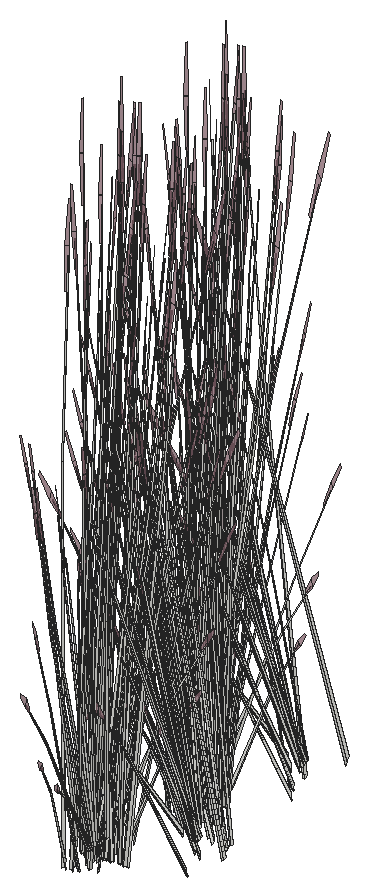
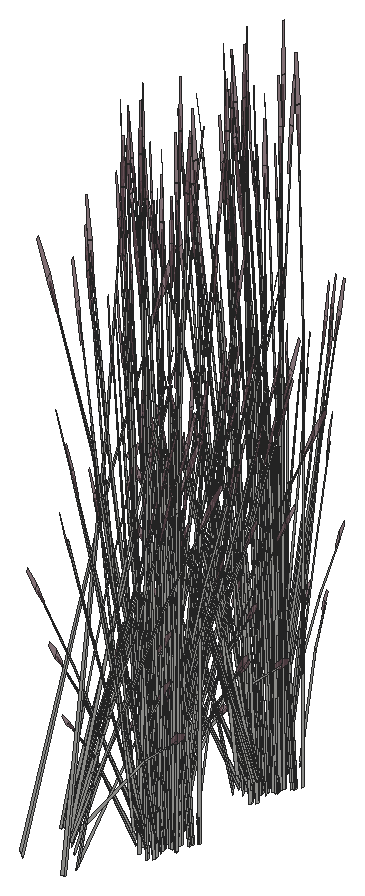
# SketchUp Ruby script. Lengths in inches.
U = 1.inch
M = Sketchup.active_model
def pt(a) = Geom::Point3d.new(a.map { |v| v * U })
def face(e, loops, mat)
  f = e.add_face(loops[0].map { |a| pt(a) })
  loops[1..].each { |l| e.add_face(l.map { |a| pt(a) }).erase! }
  f.material = f.back_material = mat if mat
  f
end
# faces: each face lists its corners as indices into pts; further lists are holes
def faces(e, pts, list, mat = nil) = list.each { |f| face(e, (f[0].is_a?(Array) ? f : [f]).map { |l| l.map { |i| pts[i] } }, mat) }
# xy, xz, yz: faces in a plane at the given z, y or x. An outline is a flat list of corners, or four numbers for a rectangle; further outlines are holes
def ring(l) = l.size == 4 ? [[l[0], l[1]], [l[2], l[1]], [l[2], l[3]], [l[0], l[3]]] : l.each_slice(2).to_a
def flat(e, list, mat, &to3) = list.each { |f| face(e, (f[0].is_a?(Array) ? f : [f]).map { |l| ring(l).map { |u, v| to3.(u, v) } }, mat) }
def xy(e, z, list, mat = nil) = flat(e, list, mat) { |x, y| [x, y, z] }
def xz(e, y, list, mat = nil) = flat(e, list, mat) { |x, z| [x, y, z] }
def yz(e, x, list, mat = nil) = flat(e, list, mat) { |y, z| [x, y, z] }
def lines(e, pts, list) = list.each { |a, b| e.add_line(pt(pts[a]), pt(pts[b])) }
# prism: a flat outline (further loops are holes) pulled along v
def prism(e, loops, v, mat = nil)
  f = face(e, loops, mat); d = Geom::Vector3d.new(v.map { |x| x * U })
  f.pushpull(f.normal.samedirection?(d) ? d.length : -d.length)
end
def box(e, o, s, mat = nil) = prism(e, [[o, [o[0] + s[0], o[1], o[2]], [o[0] + s[0], o[1] + s[1], o[2]], [o[0], o[1] + s[1], o[2]]]], [0, 0, s[2]], mat)
def at(x, y, z, deg = 0) = Geom::Transformation.translation(pt([x, y, z])) * Geom::Transformation.rotation(ORIGIN, Z_AXIS, deg.degrees)
def axes(o, x, y, z) = Geom::Transformation.new([*x, 0, *y, 0, *z, 0, *pt(o).to_a, 1])
def part(name) = M.definitions.add(name)
# library, detail: a bought-in or finely detailed component or shape, given as its bounding box
def library(name, o, s) = part(name).tap { |d| box(d.entities, o, s) }
def detail(e, o, s) = box(e.add_group.entities, o, s)
def put(e, d, t, mat = nil) = e.add_instance(d, t).tap { |i| i.material = mat if mat }
def group(e, t, mat = nil) = e.add_group.tap { |g| g.transformation = t; g.material = mat if mat }.entities
root = M.entities
M.materials.add("LightPink_Translucent").color = [144, 107, 117]
M.materials["LightPink_Translucent"].alpha = 0.75
c1 = part("blade")
p = [[2.15,0.21,22],[0,0.17,0],[0.09,0.45,0],[2.18,0.31,22],[2.29,0.31,22],[0.38,0.45,0],
  [2.48,0.24,33],[2.49,0.24,33],[2.48,0.22,33]]
faces(c1.entities,p,[[0,1,2,3],[4,5,2,3],[6,3,4,7],[8,0,3,6]])
c2 = part("seeds")
p = [[0.3,-0.1,1.38],[-0.01,-0.03,1.59],[-0.01,-0.03,0.03],[0.14,-0.07,-0.07],[0.29,-0.03,3],[0.15,0.01,3.11]]
faces(c2.entities,p,[[0,1,2,3],[1,0,4,5]],"LightPink_Translucent")
c3 = part("blade with seeds")
put(c3.entities,c1,at(0,0,0))
put(c3.entities,c2,axes([2.4,0.25,30.99],[1.5799,-0.05474,1.17369],[-0.12525,1.92788,0.29478],[-0.07173,-0.02425,1.56792]))
put(root,c3,axes([404.3,9.67,-9.59],[-0.14537,0.11002,1.33163],[-0.43536,-0.19256,-0.28638],[0.0807,-0.23948,0.56934]))
put(root,c3,axes([404.65,10.49,-7.36],[0.01331,-0.50278,-0.66157],[0.56035,0.03377,0.07984],[0.05914,-0.213,0.93586]))
put(root,c3,axes([405.43,9.7,-7.61],[-0.00494,-0.10818,1.62908],[-0.41695,-0.31265,-0.25764],[0.06446,-0.18952,0.13065]))
put(root,c3,axes([404.02,10.23,-8.39],[-0.09522,0.18683,1.59586],[-0.39947,-0.38663,0.12904],[0.18021,-0.24097,0.68222]))
put(root,c3,axes([405.32,9.32,-7.62],[-0.05194,0.04152,1.65179],[-0.50886,-0.14007,-0.15608],[-0.01842,-0.18118,0.29231]))
put(root,c3,axes([403.76,8.8,-9.42],[0.06561,0.31695,1.06958],[-0.36394,-0.17555,0.78586],[0.03916,-0.16229,0.23558]))
put(root,c3,axes([404.54,10.32,-7.64],[-0.3661,-0.36521,-0.47583],[0.38674,-0.31985,-0.36857],[0.0557,-0.18556,0.91046]))
put(root,c3,axes([403.74,9.78,-7.59],[0.50393,0.1421,0.447],[-0.17232,0.46717,0.36857],[-0.03028,-0.18372,0.92496]))
put(root,c3,axes([404.92,10.51,-7.3125],[-0.56206,-0.02693,-0.11324],[0.01536,-0.50991,-0.62851],[0.03904,-0.19638,0.95501]))
put(root,c3,axes([404.88,10.1875,-7.78],[0.34603,-0.28618,-0.32977],[0.32756,0.32677,0.42575],[0.04984,-0.16603,0.81462]))
put(root,c3,axes([404.88,10.3,-7.59],[0.36417,0.37086,0.447],[-0.38674,0.31985,0.36857],[0.06718,-0.174,0.92496]))
put(root,c3,axes([405.01,10.33,-7.6],[0.42027,0.02533,0.05988],[-0.01152,0.38243,0.47138],[0.04398,-0.14649,0.71878]))
put(root,c3,axes([404.7,10.59,-7.3],[-0.34603,0.28618,0.32977],[-0.32756,-0.32677,-0.42575],[0.04984,-0.16603,0.81462]))
put(root,c3,axes([402.42,10.12,-9.79],[-0.31974,-0.54466,0],[0.53494,-0.30375,-0.48057],[0.12184,-0.06918,1.52448]))
put(root,c3,axes([402.86,10.03,-10.12],[0.47863,-0.27177,-0.46235],[0.28609,0.48733,0],[0.10901,-0.0619,1.46668]))
put(root,c3,axes([403.42,11.15,-10.08],[0.34446,-0.40855,-0.58063],[0.42791,0.37046,-0.15239],[0.13803,-0.10191,1.28164]))
put(root,c3,axes([403.05,11.62,-9.52],[-0.05959,-0.62022,-0.27094],[0.62068,-0.0375,-0.46562],[0.1093,-0.08261,1.4872]))
put(root,c3,axes([405.3,11.48,-7.3],[-0.44516,0.07768,0.32977],[-0.11755,-0.44407,-0.42575],[0.12757,-0.11927,0.81462]))
put(root,c3,axes([402.97,10.25,-10.11],[0.47712,0.13449,-0.28847],[-0.12013,0.47362,0.28847],[0.09619,-0.05462,1.29413]))
put(root,c3,axes([403.13,12.1,-9.73],[0.57623,0.26344,0.22409],[-0.27732,0.5474,0.46562],[0,-0.12618,1.49497]))
put(root,c3,axes([402.95,11.74,-9.47],[-0.55535,0.03355,0.41661],[-0.05022,-0.55698,-0.2005],[0.09942,-0.05645,1.33761]))
put(root,c3,axes([403.73,11.99,-9.95],[0,-0.62892,0],[0.63949,0,0],[0,0,1.6711]))
put(root,c3,axes([404.5,10.54,-9.69],[-0.47863,-0.27177,0.46235],[0.28609,-0.48733,0],[0.10901,0.0619,1.46668]))
put(root,c3,axes([403.42,11.59,-9.8],[-0.42403,0.49328,0.42607],[-0.50377,-0.43543,0.16719],[0.10223,-0.04923,1.47927]))
put(root,c3,axes([402.6875,10.78,-9.7],[-0.14774,0.54019,0.16428],[-0.54062,-0.15287,0.32672],[0.09339,-0.00263,1.49371]))
put(root,c3,axes([403.82,11.38,-9.5625],[0.09866,-0.48509,0.13483],[0.48202,0.0842,-0.38503],[0.08772,0.04981,1.18024]))
put(root,c3,axes([403.61,11.51,-9.47],[-0.30722,-0.45622,0.41661],[0.46535,-0.32126,-0.2005],[0.09942,0.05645,1.33761]))
put(root,c3,axes([403.77,11.54,-9.52],[0.51635,-0.36087,-0.27094],[0.34336,0.5099,-0.46562],[0.1274,0.05178,1.4872]))
put(root,c3,axes([410.18,15.48,-7.36],[-0.43608,-0.26272,-0.66157],[0.30991,-0.46038,0.07984],[-0.158,-0.15687,0.93586]))
put(root,c3,axes([404.16,12.13,-9.95],[0.57217,0,0],[0,0.56272,0],[0,0,1.66132]))
put(root,c3,axes([404.32,10.8125,-9.7],[-0.54955,0.14427,0.16428],[-0.1357,-0.53689,0.32672],[0.04901,0.07823,1.49371]))
put(root,c3,axes([404.9375,10.78,-10.11],[0.12013,0.47362,-0.28847],[-0.47712,0.13449,0.28847],[0.09619,0.05462,1.29413]))
put(root,c3,axes([409.32,15.04,-10.61],[-0.04954,0.0716,1.6421],[-0.50062,0.15438,-0.25086],[-0.12094,-0.14044,0.2797]))
put(root,c3,axes([403.98,11.84,-9.78],[-0.64638,-0.11452,0.45814],[0.13155,-0.64678,0.17978],[0.09446,0.06245,1.59061]))
put(root,c3,axes([409.06,15.77,-8.39],[0.18996,0.09365,1.59586],[-0.39312,0.39287,0.12904],[-0.24502,-0.17723,0.68222]))
put(root,c3,axes([404.08,13.375,-9.97],[0.53691,-0.18442,-0.17877],[0.18866,0.53125,0.00007],[0.05927,-0.02038,1.61933]))
put(root,c3,axes([404.15,12.37,-9.9375],[0.35699,0.35109,0],[-0.35699,0.35109,0],[0,0,1.57621]))
put(root,c3,axes([405.11,12.22,-9.7],[-0.40181,-0.39593,0.16428],[0.40492,-0.38402,0.32672],[-0.04438,0.08086,1.49371]))
put(root,c3,axes([409.97,15.49,-7.64],[-0.50465,0.12921,-0.47583],[-0.08828,-0.48932,-0.36857],[-0.13555,-0.14022,0.91046]))
put(root,c3,axes([410.33,15.05,-6.94],[-0.34131,0.52108,-0.12682],[-0.49429,-0.3002,-0.70393],[-0.17182,-0.14722,1.06961]))
put(root,c3,axes([404.14,11.96,-9.47],[0.24813,-0.48978,0.41661],[0.51557,0.23571,-0.2005],[0,0.1129,1.33761]))
put(root,c3,axes([404.05,12.24,-9.87],[0,0.62861,-0.05249],[-0.63949,0,0],[0,0.01975,1.67027]))
put(root,c3,axes([404.09,11.8,-9.94],[0.30722,0.45622,-0.41661],[-0.46535,0.32126,0.2005],[0.09942,0.05645,1.33761]))
put(root,c3,axes([409.02,14.9,-7.61],[-0.11004,-0.00384,1.62908],[-0.35032,0.38367,-0.25764],[-0.18692,-0.07839,0.13065]))
put(root,c3,axes([405.45,12.23,-9.69],[0,-0.54355,0.46235],[0.57217,0,0],[0,0.1238,1.46668]))
put(root,c3,axes([404.36,12.07,-9.5625],[0.47648,-0.15851,0.13483],[0.16686,0.45265,-0.38503],[0,0.09962,1.18024]))
put(root,c3,axes([408.9375,15.77,-7.26],[0.42234,-0.40113,0.50064],[0.36424,0.42599,0.4128],[-0.19815,-0.07399,1.03595]))
put(root,c3,axes([403.93,13.66,-9.95],[0.51557,0.24403,0],[-0.24813,0.50705,0],[0,0,1.62917]))
put(root,c3,axes([409.13,15.77,-7.6],[0.02575,-0.41332,0.05988],[0.38885,0.01133,0.47138],[-0.14895,-0.04325,0.71878]))
put(root,c3,axes([408.98,15.9,-7.78],[-0.29098,-0.34031,-0.32977],[0.33226,-0.32215,0.42575],[-0.16881,-0.04902,0.81462]))
put(root,c3,axes([408.88,16.26,-9.59],[0.09985,0.15133,1.33163],[-0.23008,0.41134,-0.28638],[-0.23625,-0.09832,0.56934]))
put(root,c3,axes([403.74,13.46,-9.87],[0.22235,0.62444,-0.05599],[-0.63531,0.21881,0],[0.00776,0.02181,1.60327]))
put(root,c3,axes([409.29,16.125,-7.36],[-0.51122,-0.01309,-0.66157],[0.03434,-0.5511,0.07984],[-0.21658,-0.05816,0.93586]))
put(root,c3,axes([405.83,12.33,-9.79],[0.63949,0,0],[0,0.60749,-0.48057],[0,0.13836,1.52448]))
put(root,c3,axes([405.58,12.64,-9.95],[-0.63917,-0.00435,-0.04634],[0,-0.60749,0.46507],[-0.02009,0.13829,1.47457]))
put(root,c3,axes([404.2,12.11,-9.52],[0.57594,0.25935,-0.27094],[-0.27732,0.5474,-0.46562],[0.0181,0.1344,1.4872]))
put(root,c3,axes([405.45,12.73,-10.11],[-0.35699,0.33913,-0.28847],[-0.35699,-0.33913,0.28847],[0,0.10923,1.29413]))
put(root,c3,axes([408.6,15.23,-7.62],[0.03791,0.05424,1.65179],[-0.18278,0.48761,-0.15608],[-0.18511,0.00353,0.29231]))
put(root,c3,axes([409.12,16.24,-7.64],[-0.37135,0.36005,-0.47583],[-0.32522,-0.38035,-0.36857],[-0.18868,-0.05478,0.91046]))
put(root,c3,axes([403.99,14.09,-7.3],[-0.07899,-0.43781,0.32977],[0.45153,-0.11561,-0.42575],[0.12128,0.12546,0.81462]))
put(root,c3,axes([409.4,16.08,-7.3],[0.29098,0.34031,0.32977],[-0.33226,0.32215,-0.42575],[-0.16881,-0.04902,0.81462]))
put(root,c3,axes([405.69,12.74,-10.12],[0,0.54355,-0.46235],[-0.57217,0,0],[0,0.1238,1.46668]))
put(root,c3,axes([408.28,16.72,-9.42],[0.3265,-0.03889,1.06958],[-0.20711,0.3427,0.78586],[-0.16135,-0.05141,0.23558]))
put(root,c3,axes([404.3,11.57,-7.83],[-0.44191,-0.28242,1.28769],[0.46662,-0.43971,0.5556],[0.14258,0.26499,1.24467]))
put(root,c3,axes([409.32,15.86,-7.3125],[-0.02738,0.55277,-0.11324],[-0.51847,-0.01511,-0.62851],[-0.19968,-0.0384,0.95501]))
put(root,c3,axes([404.96,13.87,-9.42],[-0.28795,-0.15629,1.06958],[0.37181,-0.1588,0.78586],[0.10029,0.13452,0.23558]))
put(root,c3,axes([404.92,20.27,-9.59],[-0.14537,0.11002,1.33163],[-0.43536,-0.19256,-0.28638],[0.0807,-0.23948,0.56934]))
put(root,c3,axes([403.55,14.7,-7.62],[0.00151,-0.06581,1.65179],[0.43826,-0.29033,-0.15608],[0.15223,0.10363,0.29231]))
put(root,c3,axes([404.43,12.66,-10.05],[0.18752,0.49766,-0.6445],[-0.54017,0.17923,-0.16915],[0.02073,0.16852,1.42262]))
put(root,c3,axes([405.27,21.09,-7.36],[0.01331,-0.50278,-0.66157],[0.56035,0.03377,0.07984],[0.05914,-0.213,0.93586]))
put(root,c3,axes([410.23,18.05,-10.08],[-0.53199,-0.08911,-0.58063],[0.11226,-0.54969,-0.15239],[-0.15876,-0.06661,1.28164]))
put(root,c3,axes([402.91,14.15,-7.3],[0.15418,-0.41799,0.32977],[0.44981,0.12192,-0.42575],[0.04124,0.16829,0.81462]))
put(root,c3,axes([406.05,20.3,-7.61],[-0.00494,-0.10818,1.62908],[-0.41695,-0.31265,-0.25764],[0.06446,-0.18952,0.13065]))
put(root,c3,axes([404.3,20.28,-7.78],[0.15418,-0.41799,-0.32977],[0.44981,0.12192,0.42575],[-0.04124,-0.16829,0.81462]))
put(root,c3,axes([405.9375,19.91,-7.62],[-0.05194,0.04152,1.65179],[-0.50886,-0.14007,-0.15608],[-0.01842,-0.18118,0.29231]))
put(root,c3,axes([405.01,14.58,-9.52],[-0.32795,-0.01705,0.97832],[0.21658,-0.36206,0.54015],[0.12956,0.12863,0.76741]))
put(root,c3,axes([404.38,19.4,-9.42],[0.06561,0.31695,1.06958],[-0.36394,-0.17555,0.78586],[0.03916,-0.16229,0.23558]))
put(root,c3,axes([408.57,17.03,-7.59],[0.14449,-0.4956,0.447],[0.47502,0.16947,0.36857],[-0.1868,0.02978,0.92496]))
put(root,c3,axes([404.07,14.48,-7.6],[-0.23243,0.34529,0.05988],[-0.331,-0.20103,0.47138],[0.10701,0.1107,0.71878]))
put(root,c3,axes([405.16,20.92,-7.64],[-0.3661,-0.36521,-0.47583],[0.38674,-0.31985,-0.36857],[0.0557,-0.18556,0.91046]))
put(root,c3,axes([408.53,16.89,-7.6],[-0.18783,-0.37061,0.05988],[0.34252,-0.1814,0.47138],[-0.15099,0.03579,0.71878]))
put(root,c3,axes([403.52,15.65,-6.74],[0.35341,-0.31182,-0.06041],[0.32382,0.34152,-0.27392],[0.0228,0.09677,0.90349]))
put(root,c3,axes([404.16,14.39,-7.59],[-0.50866,0.12474,0.447],[-0.08828,-0.48932,0.36857],[0.11963,0.14421,0.92496]))
put(root,c3,axes([408.52,17.28,-10.61],[0.01297,0.08566,1.6421],[-0.26146,0.44735,-0.25086],[-0.18572,-0.02255,0.2797]))
put(root,c3,axes([403.9375,13.7,-9.59],[0.00902,-0.18018,1.33163],[0.43127,-0.20126,-0.28638],[0.13313,0.21566,0.56934]))
put(root,c3,axes([404.35,20.38,-7.59],[0.50393,0.1421,0.447],[-0.17232,0.46717,0.36857],[-0.03028,-0.18372,0.92496]))
put(root,c3,axes([405.54,21.11,-7.3125],[-0.56206,-0.02693,-0.11324],[0.01536,-0.50991,-0.62851],[0.03904,-0.19638,0.95501]))
put(root,c3,axes([405.5,20.79,-7.78],[0.34603,-0.28618,-0.32977],[0.32756,0.32677,0.42575],[0.04984,-0.16603,0.81462]))
put(root,c3,axes([404.49,20.34,-7.6],[0.37684,-0.18473,0.05988],[0.18445,0.33686,0.47138],[-0.03639,-0.14849,0.71878]))
put(root,c3,axes([409.53,19.09,-10.12],[-0.47863,-0.27177,-0.46235],[0.28609,-0.48733,0],[-0.10901,-0.0619,1.46668]))
put(root,c3,axes([402.76,14.33,-7.3125],[0.50045,-0.25306,-0.11324],[0.24593,0.44915,-0.62851],[0.06603,0.18927,0.95501]))
put(root,c3,axes([408.47,17.08,-7.78],[-0.42502,-0.15163,-0.32977],[0.12396,-0.44238,0.42575],[-0.17112,0.04056,0.81462]))
put(root,c3,axes([403.19,14.31,-7.64],[0.50273,0.13626,-0.47583],[-0.17232,0.46717,-0.36857],[0.0461,0.18809,0.91046]))
put(root,c3,axes([403.48,13.34,-8.39],[-0.1169,-0.17452,1.59586],[0.54019,-0.14692,0.12904],[0.12209,0.27397,0.68222]))
put(root,c3,axes([408.92,17.03,-7.3],[0.42502,0.15163,0.32977],[-0.12396,0.44238,-0.42575],[-0.17112,0.04056,0.81462]))
put(root,c3,axes([409.76,17.01,-8.89],[0.14537,-0.07863,1.64882],[0.05013,0.549,0.12904],[-0.31487,0.07285,0.5893]))
put(root,c3,axes([405.5,20.9,-7.59],[0.36417,0.37086,0.447],[-0.38674,0.31985,0.36857],[0.06718,-0.174,0.92496]))
put(root,c3,axes([405.63,20.93,-7.6],[0.42027,0.02533,0.05988],[-0.01152,0.38243,0.47138],[0.04398,-0.14649,0.71878]))
put(root,c3,axes([405.32,21.19,-7.3],[-0.34603,0.28618,0.32977],[-0.32756,-0.32677,-0.42575],[0.04984,-0.16603,0.81462]))
put(root,c3,axes([403.04,20.71,-9.79],[-0.31974,-0.54466,0],[0.53494,-0.30375,-0.48057],[0.12184,-0.06918,1.52448]))
put(root,c3,axes([403.01,14.22,-7.36],[0.24409,0.44196,-0.66157],[-0.50245,0.2463,0.07984],[0.05708,0.21354,0.93586]))
put(root,c3,axes([408.2,17.375,-7.61],[-0.08351,0.07057,1.62908],[0.0071,0.51561,-0.25764],[-0.19143,0.06705,0.13065]))
put(root,c3,axes([408.76,17.31,-7.64],[-0.13855,0.49442,-0.47583],[-0.47502,-0.16947,-0.36857],[-0.19125,0.04534,0.91046]))
put(root,c3,axes([408.74,16.88,-7.3125],[0.25732,0.49218,-0.11324],[-0.45669,0.24187,-0.62851],[-0.19245,0.06494,0.95501]))
put(root,c3,axes([409.83,19.42,-9.79],[-0.31974,0.54466,0],[-0.53494,-0.30375,-0.48057],[-0.12184,-0.06918,1.52448]))
put(root,c3,axes([403.48,20.63,-10.12],[0.47863,-0.27177,-0.46235],[0.28609,0.48733,0],[0.10901,-0.0619,1.46668]))
put(root,c3,axes([404.04,21.74,-10.08],[0.34446,-0.40855,-0.58063],[0.42791,0.37046,-0.15239],[0.13803,-0.10191,1.28164]))
put(root,c3,axes([408.68,18.26,-7.59],[-0.12683,-0.50025,0.447],[0.49754,-0.08682,0.36857],[-0.14663,0.11765,0.92496]))
put(root,c3,axes([408.58,18.16,-7.6],[-0.35109,-0.22859,0.05988],[0.2044,-0.32553,0.47138],[-0.11256,0.10524,0.71878]))
put(root,c3,axes([408.74,17.5625,-8.39],[0.17745,-0.11497,1.59586],[0.14939,0.53127,0.12904],[-0.27857,0.12007,0.68222]))
put(root,c3,axes([403.44,22.46,-9.94],[0.24813,-0.48978,-0.41661],[0.51557,0.23571,0.2005],[0,-0.1129,1.33761]))
put(root,c3,axes([403.67,22.22,-9.52],[-0.05959,-0.62022,-0.27094],[0.62068,-0.0375,-0.46562],[0.1093,-0.08261,1.4872]))
put(root,c3,axes([403.59,20.84,-10.11],[0.47712,0.13449,-0.28847],[-0.12013,0.47362,0.28847],[0.09619,-0.05462,1.29413]))
put(root,c3,axes([408.19,18.47,-9.59],[0.17773,0.04462,1.33163],[0.11455,0.45576,-0.28638],[-0.24142,0.08531,0.56934]))
put(root,c3,axes([407.27,17.9,-7.62],[0.06527,0.01458,1.65179],[0.20191,0.48025,-0.15608],[-0.1336,0.12605,0.29231]))
put(root,c3,axes([407.82,19.42,-9.42],[0.21313,-0.24635,1.06958],[0.0841,0.38999,0.78586],[-0.15402,0.06983,0.23558]))
put(root,c3,axes([408.625,18.36,-7.78],[-0.44516,0.07768,-0.32977],[-0.11755,-0.44407,0.42575],[-0.12757,0.11927,0.81462]))
put(root,c3,axes([403.75,22.7,-9.73],[0.57623,0.26344,0.22409],[-0.27732,0.5474,0.46562],[0,-0.12618,1.49497]))
put(root,c3,axes([403.56,22.34,-9.47],[-0.55535,0.03355,0.41661],[-0.05022,-0.55698,-0.2005],[0.09942,-0.05645,1.33761]))
put(root,c3,axes([408.76,18.05,-7.3125],[0.47307,0.29971,-0.11324],[-0.27254,0.43404,-0.62851],[-0.13365,0.15087,0.95501]))
put(root,c3,axes([403.55,22.54,-9.8],[0.22235,0.6078,0.42607],[-0.63531,0.21135,0.16719],[0.00776,-0.11168,1.47927]))
put(root,c3,axes([409.39,17.92,-8.39],[0.12773,-0.16701,1.59586],[0.32252,0.4508,0.12904],[-0.22121,0.20529,0.68222]))
put(root,c3,axes([408.99,18.41,-7.64],[0.13138,0.49631,-0.47583],[-0.49754,0.08682,-0.36857],[-0.14258,0.13331,0.91046]))
put(root,c3,axes([404.35,22.59,-9.95],[0,-0.62892,0],[0.63949,0,0],[0,0,1.6711]))
put(root,c3,axes([405.12,21.13,-9.69],[-0.47863,-0.27177,0.46235],[0.28609,-0.48733,0],[0.10901,0.0619,1.46668]))
put(root,c3,axes([408.38,19.67,-10.61],[0.0686,0.0543,1.6421],[0.11632,0.50315,-0.25086],[-0.15204,0.10729,0.2797]))
put(root,c3,axes([404.04,22.19,-9.8],[-0.42403,0.49328,0.42607],[-0.50377,-0.43543,0.16719],[0.10223,-0.04923,1.47927]))
put(root,c3,axes([403.31,21.38,-9.7],[-0.14774,0.54019,0.16428],[-0.54062,-0.15287,0.32672],[0.09339,-0.00263,1.49371]))
put(root,c3,axes([404.43,21.98,-9.5625],[0.09866,-0.48509,0.13483],[0.48202,0.0842,-0.38503],[0.08772,0.04981,1.18024]))
put(root,c3,axes([404.23,22.11,-9.47],[-0.30722,-0.45622,0.41661],[0.46535,-0.32126,-0.2005],[0.09942,0.05645,1.33761]))
put(root,c3,axes([409.3,18.33,-8.39],[0.09522,-0.18683,1.59586],[0.39947,0.38663,0.12904],[-0.18021,0.24097,0.68222]))
put(root,c3,axes([408.21,19.3,-7.61],[-0.01271,0.10756,1.62908],[0.36076,0.37419,-0.25764],[-0.09444,0.17695,0.13065]))
put(root,c3,axes([404.78,22.73,-9.95],[0.57217,0,0],[0,0.56272,0],[0,0,1.66132]))
put(root,c3,axes([404.94,21.41,-9.7],[-0.54955,0.14427,0.16428],[-0.1357,-0.53689,0.32672],[0.04901,0.07823,1.49371]))
put(root,c3,axes([408.84,27.92,-8.39],[0.1169,0.17452,1.59586],[-0.54019,0.14692,0.12904],[-0.12209,-0.27397,0.68222]))
put(root,c3,axes([404.59,22.44,-9.78],[-0.64638,-0.11452,0.45814],[0.13155,-0.64678,0.17978],[0.09446,0.06245,1.59061]))
put(root,c3,axes([404.08,24.04,-9.95],[-0.16686,-0.46861,0],[0.47648,-0.16411,0],[0,0,1.4375]))
put(root,c3,axes([404.7,23.97,-9.97],[0.53691,-0.18442,-0.17877],[0.18866,0.53125,0.00007],[0.05927,-0.02038,1.61933]))
put(root,c3,axes([404.77,22.97,-9.9375],[0.35699,0.35109,0],[-0.35699,0.35109,0],[0,0,1.57621]))
put(root,c3,axes([408.69,27.46,-9.59],[-0.03097,0.17781,1.33163],[-0.45273,0.14885,-0.28638],[-0.10583,-0.22982,0.56934]))
put(root,c3,axes([405.73,22.82,-9.7],[-0.40181,-0.39593,0.16428],[0.40492,-0.38402,0.32672],[-0.04438,0.08086,1.49371]))
put(root,c3,axes([404.76,22.56,-9.47],[0.24813,-0.48978,0.41661],[0.51557,0.23571,-0.2005],[0,0.1129,1.33761]))
put(root,c3,axes([404.67,22.84,-9.87],[0,0.62861,-0.05249],[-0.63949,0,0],[0,0.01975,1.67027]))
put(root,c3,axes([404.71,22.39,-9.94],[0.30722,0.45622,-0.41661],[-0.46535,0.32126,0.2005],[0.09942,0.05645,1.33761]))
put(root,c3,axes([406.0625,22.83,-9.69],[0,-0.54355,0.46235],[0.57217,0,0],[0,0.1238,1.46668]))
put(root,c3,axes([404.98,22.67,-9.5625],[0.47648,-0.15851,0.13483],[0.16686,0.45265,-0.38503],[0,0.09962,1.18024]))
put(root,c3,axes([409.19,26.51,-7.62],[-0.00954,0.06515,1.65179],[-0.47055,0.23645,-0.15608],[-0.13847,-0.12087,0.29231]))
put(root,c3,axes([404.55,24.26,-9.95],[0.51557,0.24403,0],[-0.24813,0.50705,0],[0,0,1.62917]))
put(root,c3,axes([409.18,28.17,-7.36],[-0.43608,-0.26272,-0.66157],[0.30991,-0.46038,0.07984],[-0.158,-0.15687,0.93586]))
put(root,c3,axes([409.03,27.83,-7.78],[-0.07899,-0.43781,-0.32977],[0.45153,-0.11561,0.42575],[-0.12128,-0.12546,0.81462]))
put(root,c3,axes([405.04,24.48,-9.69],[0.47863,-0.27177,0.46235],[0.28609,0.48733,0],[-0.10901,0.0619,1.46668]))
put(root,c3,axes([408.32,27.74,-10.61],[-0.04954,0.0716,1.6421],[-0.50062,0.15438,-0.25086],[-0.12094,-0.14044,0.2797]))
put(root,c3,axes([404.36,24.06,-9.87],[0.22235,0.62444,-0.05599],[-0.63531,0.21881,0],[0.00776,0.02181,1.60327]))
put(root,c3,axes([408.06,28.46,-8.39],[0.18996,0.09365,1.59586],[-0.39312,0.39287,0.12904],[-0.24502,-0.17723,0.68222]))
put(root,c3,axes([406.2,23.24,-9.95],[-0.63917,-0.00435,-0.04634],[0,-0.60749,0.46507],[-0.02009,0.13829,1.47457]))
put(root,c3,axes([404.8125,22.71,-9.52],[0.57594,0.25935,-0.27094],[-0.27732,0.5474,-0.46562],[0.0181,0.1344,1.4872]))
put(root,c3,axes([406.0625,23.33,-10.11],[-0.35699,0.33913,-0.28847],[-0.35699,-0.33913,0.28847],[0,0.10923,1.29413]))
put(root,c3,axes([408.97,28.1875,-7.64],[-0.50465,0.12921,-0.47583],[-0.08828,-0.48932,-0.36857],[-0.13555,-0.14022,0.91046]))
put(root,c3,axes([409.33,27.75,-6.94],[-0.34131,0.52108,-0.12682],[-0.49429,-0.3002,-0.70393],[-0.17182,-0.14722,1.06961]))
put(root,c3,axes([404.75,23.12,-9.94],[-0.24813,0.48978,-0.41661],[-0.51557,-0.23571,0.2005],[0,0.1129,1.33761]))
put(root,c3,axes([408.02,27.6,-7.61],[-0.11004,-0.00384,1.62908],[-0.35032,0.38367,-0.25764],[-0.18692,-0.07839,0.13065]))
put(root,c3,axes([404.61,24.68,-7.3],[-0.07899,-0.43781,0.32977],[0.45153,-0.11561,-0.42575],[0.12128,0.12546,0.81462]))
put(root,c3,axes([406.31,23.34,-10.12],[0,0.54355,-0.46235],[-0.57217,0,0],[0,0.1238,1.46668]))
put(root,c3,axes([404.92,22.17,-7.83],[-0.44191,-0.28242,1.28769],[0.46662,-0.43971,0.5556],[0.14258,0.26499,1.24467]))
put(root,c3,axes([410.22,31.15,-8.9],[0.44194,0.21918,1.40854],[-0.43295,0.47219,0.557],[-0.19393,-0.27986,1.18082]))
put(root,c3,axes([409.29,28.18,-7.3],[0.07899,0.43781,0.32977],[-0.45153,0.11561,-0.42575],[-0.12128,-0.12546,0.81462]))
put(root,c3,axes([407.9375,28.47,-7.26],[0.42234,-0.40113,0.50064],[0.36424,0.42599,0.4128],[-0.19815,-0.07399,1.03595]))
put(root,c3,axes([405.58,24.46,-9.42],[-0.28795,-0.15629,1.06958],[0.37181,-0.1588,0.78586],[0.10029,0.13452,0.23558]))
put(root,c3,axes([404.17,25.3,-7.62],[0.00151,-0.06581,1.65179],[0.43826,-0.29033,-0.15608],[0.15223,0.10363,0.29231]))
put(root,c3,axes([405.04,23.26,-10.05],[0.18752,0.49766,-0.6445],[-0.54017,0.17923,-0.16915],[0.02073,0.16852,1.42262]))
put(root,c3,axes([408.13,28.47,-7.6],[0.02575,-0.41332,0.05988],[0.38885,0.01133,0.47138],[-0.14895,-0.04325,0.71878]))
put(root,c3,axes([407.98,28.6,-7.78],[-0.29098,-0.34031,-0.32977],[0.33226,-0.32215,0.42575],[-0.16881,-0.04902,0.81462]))
put(root,c3,axes([403.53,24.75,-7.3],[0.15418,-0.41799,0.32977],[0.44981,0.12192,-0.42575],[0.04124,0.16829,0.81462]))
put(root,c3,axes([408.01,28.02,-10.02],[-0.14753,0.44383,-0.03625],[-0.45406,-0.13653,-0.16435],[-0.06894,-0.07259,0.54209]))
put(root,c3,axes([407.77,30.04,-9.79],[-0.63949,0,0],[0,-0.60749,-0.48057],[0,-0.13836,1.52448]))
put(root,c3,axes([404.68,25.08,-7.6],[-0.23243,0.34529,0.05988],[-0.331,-0.20103,0.47138],[0.10701,0.1107,0.71878]))
put(root,c3,axes([404.14,26.24,-6.74],[0.35341,-0.31182,-0.06041],[0.32382,0.34152,-0.27392],[0.0228,0.09677,0.90349]))
put(root,c3,axes([404.78,24.98,-7.59],[-0.50866,0.12474,0.447],[-0.08828,-0.48932,0.36857],[0.11963,0.14421,0.92496]))
put(root,c3,axes([404.56,24.3,-9.59],[0.00902,-0.18018,1.33163],[0.43127,-0.20126,-0.28638],[0.13313,0.21566,0.56934]))
